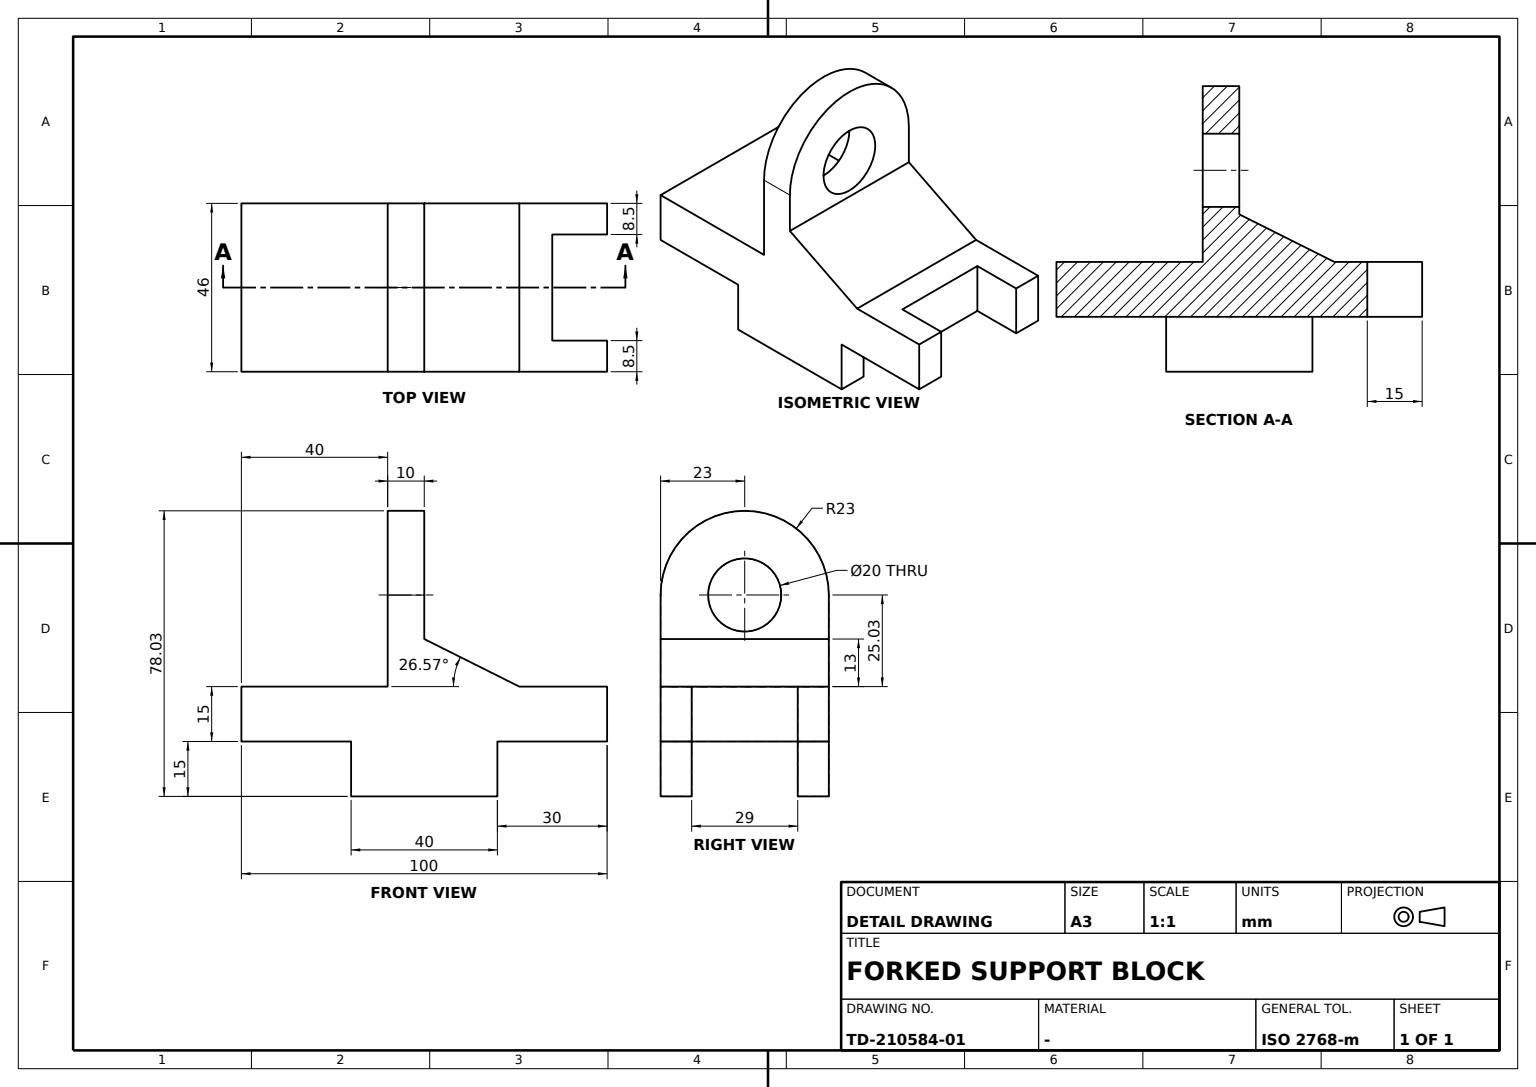
ISO-10303-21;
HEADER;
FILE_DESCRIPTION((''),'2;1');
FILE_NAME('','',(''),(''),'','','');
FILE_SCHEMA(('AUTOMOTIVE_DESIGN'));
ENDSEC;
DATA;
#1=APPLICATION_CONTEXT('');
#2=PRODUCT_CONTEXT('',#1,'mechanical');
#3=PRODUCT('','','',(#2));
#4=PRODUCT_DEFINITION_FORMATION('','',#3);
#5=PRODUCT_DEFINITION_CONTEXT('',#1,'design');
#6=PRODUCT_DEFINITION('','',#4,#5);
#7=PRODUCT_DEFINITION_SHAPE('','',#6);
#8=(LENGTH_UNIT()NAMED_UNIT(*)SI_UNIT(.MILLI.,.METRE.));
#9=(NAMED_UNIT(*)PLANE_ANGLE_UNIT()SI_UNIT($,.RADIAN.));
#10=(NAMED_UNIT(*)SI_UNIT($,.STERADIAN.)SOLID_ANGLE_UNIT());
#11=UNCERTAINTY_MEASURE_WITH_UNIT(LENGTH_MEASURE(1.E-05),#8,'distance_accuracy_value','');
#12=(GEOMETRIC_REPRESENTATION_CONTEXT(3)GLOBAL_UNCERTAINTY_ASSIGNED_CONTEXT((#11))GLOBAL_UNIT_ASSIGNED_CONTEXT((#8,#9,#10))REPRESENTATION_CONTEXT('',''));
#13=CARTESIAN_POINT('',(-20.,14.5,0.));
#14=VERTEX_POINT('',#13);
#15=CARTESIAN_POINT('',(-20.,23.,0.));
#16=VERTEX_POINT('',#15);
#17=CARTESIAN_POINT('',(-20.,18.75,0.));
#18=DIRECTION('',(0.,1.,0.));
#19=VECTOR('',#18,1000.);
#20=LINE('',#17,#19);
#21=EDGE_CURVE('',#14,#16,#20,.T.);
#22=ORIENTED_EDGE('',*,*,#21,.T.);
#23=CARTESIAN_POINT('',(20.,23.,0.));
#24=VERTEX_POINT('',#23);
#25=CARTESIAN_POINT('',(0.,23.,0.));
#26=DIRECTION('',(-1.,0.,0.));
#27=VECTOR('',#26,1000.);
#28=LINE('',#25,#27);
#29=EDGE_CURVE('',#24,#16,#28,.T.);
#30=ORIENTED_EDGE('',*,*,#29,.F.);
#31=CARTESIAN_POINT('',(20.,14.5,0.));
#32=VERTEX_POINT('',#31);
#33=CARTESIAN_POINT('',(20.,18.75,0.));
#34=LINE('',#33,#19);
#35=EDGE_CURVE('',#32,#24,#34,.T.);
#36=ORIENTED_EDGE('',*,*,#35,.F.);
#37=CARTESIAN_POINT('',(0.,14.5,0.));
#38=DIRECTION('',(1.,0.,0.));
#39=VECTOR('',#38,1000.);
#40=LINE('',#37,#39);
#41=EDGE_CURVE('',#14,#32,#40,.T.);
#42=ORIENTED_EDGE('',*,*,#41,.F.);
#43=EDGE_LOOP('',(#22,#30,#36,#42));
#44=FACE_OUTER_BOUND('',#43,.T.);
#45=CARTESIAN_POINT('',(20.,0.,0.));
#46=DIRECTION('',(0.,0.,-1.));
#47=AXIS2_PLACEMENT_3D('',#45,#46,#26);
#48=PLANE('',#47);
#49=ADVANCED_FACE('',(#44),#48,.T.);
#50=CARTESIAN_POINT('',(-20.,14.5,15.));
#51=VERTEX_POINT('',#50);
#52=CARTESIAN_POINT('',(-20.,23.,15.));
#53=VERTEX_POINT('',#52);
#54=CARTESIAN_POINT('',(-20.,18.75,15.));
#55=LINE('',#54,#19);
#56=EDGE_CURVE('',#51,#53,#55,.T.);
#57=ORIENTED_EDGE('',*,*,#56,.T.);
#58=CARTESIAN_POINT('',(-20.,23.,7.5));
#59=DIRECTION('',(0.,0.,1.));
#60=VECTOR('',#59,1000.);
#61=LINE('',#58,#60);
#62=EDGE_CURVE('',#16,#53,#61,.T.);
#63=ORIENTED_EDGE('',*,*,#62,.F.);
#64=ORIENTED_EDGE('',*,*,#21,.F.);
#65=CARTESIAN_POINT('',(-20.,14.5,7.5));
#66=VECTOR('',#46,1000.);
#67=LINE('',#65,#66);
#68=EDGE_CURVE('',#51,#14,#67,.T.);
#69=ORIENTED_EDGE('',*,*,#68,.F.);
#70=EDGE_LOOP('',(#57,#63,#64,#69));
#71=FACE_OUTER_BOUND('',#70,.T.);
#72=CARTESIAN_POINT('',(-20.,0.,0.));
#73=AXIS2_PLACEMENT_3D('',#72,#26,#59);
#74=PLANE('',#73);
#75=ADVANCED_FACE('',(#71),#74,.T.);
#76=CARTESIAN_POINT('',(50.,14.5,15.));
#77=VERTEX_POINT('',#76);
#78=CARTESIAN_POINT('',(50.,23.,15.));
#79=VERTEX_POINT('',#78);
#80=CARTESIAN_POINT('',(50.,18.75,15.));
#81=LINE('',#80,#19);
#82=EDGE_CURVE('',#77,#79,#81,.T.);
#83=ORIENTED_EDGE('',*,*,#82,.T.);
#84=CARTESIAN_POINT('',(50.,23.,30.));
#85=VERTEX_POINT('',#84);
#86=CARTESIAN_POINT('',(50.,23.,22.5));
#87=LINE('',#86,#66);
#88=EDGE_CURVE('',#85,#79,#87,.T.);
#89=ORIENTED_EDGE('',*,*,#88,.F.);
#90=CARTESIAN_POINT('',(50.,14.5,30.));
#91=VERTEX_POINT('',#90);
#92=CARTESIAN_POINT('',(50.,18.75,30.));
#93=LINE('',#92,#19);
#94=EDGE_CURVE('',#91,#85,#93,.T.);
#95=ORIENTED_EDGE('',*,*,#94,.F.);
#96=CARTESIAN_POINT('',(50.,14.5,22.5));
#97=LINE('',#96,#66);
#98=EDGE_CURVE('',#91,#77,#97,.T.);
#99=ORIENTED_EDGE('',*,*,#98,.T.);
#100=EDGE_LOOP('',(#83,#89,#95,#99));
#101=FACE_OUTER_BOUND('',#100,.T.);
#102=CARTESIAN_POINT('',(50.,0.,15.));
#103=AXIS2_PLACEMENT_3D('',#102,#26,#59);
#104=PLANE('',#103);
#105=ADVANCED_FACE('',(#101),#104,.F.);
#106=CARTESIAN_POINT('',(-10.,23.,55.034304));
#107=VERTEX_POINT('',#106);
#108=CARTESIAN_POINT('',(-10.,-23.,55.034304));
#109=VERTEX_POINT('',#108);
#110=CARTESIAN_POINT('',(-10.,0.,55.034304));
#111=AXIS2_PLACEMENT_3D('',#110,#38,#18);
#112=CIRCLE('',#111,23.);
#113=EDGE_CURVE('',#107,#109,#112,.T.);
#114=ORIENTED_EDGE('',*,*,#113,.F.);
#115=CARTESIAN_POINT('',(-10.,23.,55.));
#116=VERTEX_POINT('',#115);
#117=EDGE_CURVE('',#116,#107,#112,.T.);
#118=ORIENTED_EDGE('',*,*,#117,.F.);
#119=CARTESIAN_POINT('',(-10.,23.,30.));
#120=VERTEX_POINT('',#119);
#121=CARTESIAN_POINT('',(-10.,23.,42.5));
#122=LINE('',#121,#60);
#123=EDGE_CURVE('',#120,#116,#122,.T.);
#124=ORIENTED_EDGE('',*,*,#123,.F.);
#125=CARTESIAN_POINT('',(-10.,-23.,30.));
#126=VERTEX_POINT('',#125);
#127=CARTESIAN_POINT('',(-10.,0.,30.));
#128=LINE('',#127,#19);
#129=EDGE_CURVE('',#126,#120,#128,.T.);
#130=ORIENTED_EDGE('',*,*,#129,.F.);
#131=CARTESIAN_POINT('',(-10.,-22.999974,55.));
#132=VERTEX_POINT('',#131);
#133=CARTESIAN_POINT('',(-10.,-23.,42.5));
#134=LINE('',#133,#60);
#135=EDGE_CURVE('',#126,#132,#134,.T.);
#136=ORIENTED_EDGE('',*,*,#135,.T.);
#137=EDGE_CURVE('',#109,#132,#112,.T.);
#138=ORIENTED_EDGE('',*,*,#137,.F.);
#139=EDGE_LOOP('',(#114,#118,#124,#130,#136,#138));
#140=FACE_OUTER_BOUND('',#139,.T.);
#141=CARTESIAN_POINT('',(-10.,-10.,55.034304));
#142=VERTEX_POINT('',#141);
#143=CARTESIAN_POINT('',(-10.,10.,55.034304));
#144=VERTEX_POINT('',#143);
#145=CIRCLE('',#111,10.);
#146=EDGE_CURVE('',#142,#144,#145,.T.);
#147=ORIENTED_EDGE('',*,*,#146,.T.);
#148=EDGE_CURVE('',#144,#142,#145,.T.);
#149=ORIENTED_EDGE('',*,*,#148,.T.);
#150=EDGE_LOOP('',(#147,#149));
#151=FACE_BOUND('',#150,.T.);
#152=AXIS2_PLACEMENT_3D('',#127,#26,#59);
#153=PLANE('',#152);
#154=ADVANCED_FACE('',(#140,#151),#153,.T.);
#155=CARTESIAN_POINT('',(-20.,-14.5,0.));
#156=VERTEX_POINT('',#155);
#157=CARTESIAN_POINT('',(20.,-14.5,0.));
#158=VERTEX_POINT('',#157);
#159=CARTESIAN_POINT('',(0.,-14.5,0.));
#160=LINE('',#159,#39);
#161=EDGE_CURVE('',#156,#158,#160,.T.);
#162=ORIENTED_EDGE('',*,*,#161,.F.);
#163=CARTESIAN_POINT('',(-20.,-14.5,15.));
#164=VERTEX_POINT('',#163);
#165=CARTESIAN_POINT('',(-20.,-14.5,7.5));
#166=LINE('',#165,#60);
#167=EDGE_CURVE('',#156,#164,#166,.T.);
#168=ORIENTED_EDGE('',*,*,#167,.T.);
#169=CARTESIAN_POINT('',(20.,-14.5,15.));
#170=VERTEX_POINT('',#169);
#171=CARTESIAN_POINT('',(0.,-14.5,15.));
#172=LINE('',#171,#39);
#173=EDGE_CURVE('',#164,#170,#172,.T.);
#174=ORIENTED_EDGE('',*,*,#173,.T.);
#175=CARTESIAN_POINT('',(20.,-14.5,7.5));
#176=LINE('',#175,#66);
#177=EDGE_CURVE('',#170,#158,#176,.T.);
#178=ORIENTED_EDGE('',*,*,#177,.T.);
#179=EDGE_LOOP('',(#162,#168,#174,#178));
#180=FACE_OUTER_BOUND('',#179,.T.);
#181=DIRECTION('',(0.,-1.,0.));
#182=AXIS2_PLACEMENT_3D('',#163,#181,#46);
#183=PLANE('',#182);
#184=ADVANCED_FACE('',(#180),#183,.F.);
#185=CARTESIAN_POINT('',(35.,14.5,15.));
#186=VERTEX_POINT('',#185);
#187=CARTESIAN_POINT('',(42.5,14.5,15.));
#188=LINE('',#187,#27);
#189=EDGE_CURVE('',#77,#186,#188,.T.);
#190=ORIENTED_EDGE('',*,*,#189,.F.);
#191=ORIENTED_EDGE('',*,*,#98,.F.);
#192=CARTESIAN_POINT('',(35.,14.5,30.));
#193=VERTEX_POINT('',#192);
#194=CARTESIAN_POINT('',(42.5,14.5,30.));
#195=LINE('',#194,#27);
#196=EDGE_CURVE('',#91,#193,#195,.T.);
#197=ORIENTED_EDGE('',*,*,#196,.T.);
#198=CARTESIAN_POINT('',(35.,14.5,22.5));
#199=LINE('',#198,#66);
#200=EDGE_CURVE('',#193,#186,#199,.T.);
#201=ORIENTED_EDGE('',*,*,#200,.T.);
#202=EDGE_LOOP('',(#190,#191,#197,#201));
#203=FACE_OUTER_BOUND('',#202,.T.);
#204=AXIS2_PLACEMENT_3D('',#13,#18,#59);
#205=PLANE('',#204);
#206=ADVANCED_FACE('',(#203),#205,.F.);
#207=CARTESIAN_POINT('',(0.,23.,55.034304));
#208=VERTEX_POINT('',#207);
#209=CARTESIAN_POINT('',(-5.,23.,55.034304));
#210=LINE('',#209,#27);
#211=EDGE_CURVE('',#208,#107,#210,.T.);
#212=ORIENTED_EDGE('',*,*,#211,.T.);
#213=ORIENTED_EDGE('',*,*,#113,.T.);
#214=CARTESIAN_POINT('',(0.,-23.,55.034304));
#215=VERTEX_POINT('',#214);
#216=CARTESIAN_POINT('',(-5.,-23.,55.034304));
#217=LINE('',#216,#27);
#218=EDGE_CURVE('',#215,#109,#217,.T.);
#219=ORIENTED_EDGE('',*,*,#218,.F.);
#220=CARTESIAN_POINT('',(0.,0.,55.034304));
#221=AXIS2_PLACEMENT_3D('',#220,#38,#18);
#222=CIRCLE('',#221,23.);
#223=EDGE_CURVE('',#208,#215,#222,.T.);
#224=ORIENTED_EDGE('',*,*,#223,.F.);
#225=EDGE_LOOP('',(#212,#213,#219,#224));
#226=FACE_OUTER_BOUND('',#225,.T.);
#227=CARTESIAN_POINT('',(-5.,0.,55.034304));
#228=AXIS2_PLACEMENT_3D('',#227,#26,#18);
#229=CYLINDRICAL_SURFACE('',#228,23.);
#230=ADVANCED_FACE('',(#226),#229,.T.);
#231=CARTESIAN_POINT('',(20.,-23.,0.));
#232=VERTEX_POINT('',#231);
#233=CARTESIAN_POINT('',(20.,-18.75,0.));
#234=LINE('',#233,#19);
#235=EDGE_CURVE('',#232,#158,#234,.T.);
#236=ORIENTED_EDGE('',*,*,#235,.F.);
#237=CARTESIAN_POINT('',(-20.,-23.,0.));
#238=VERTEX_POINT('',#237);
#239=CARTESIAN_POINT('',(0.,-23.,0.));
#240=LINE('',#239,#27);
#241=EDGE_CURVE('',#232,#238,#240,.T.);
#242=ORIENTED_EDGE('',*,*,#241,.T.);
#243=CARTESIAN_POINT('',(-20.,-18.75,0.));
#244=LINE('',#243,#19);
#245=EDGE_CURVE('',#238,#156,#244,.T.);
#246=ORIENTED_EDGE('',*,*,#245,.T.);
#247=ORIENTED_EDGE('',*,*,#161,.T.);
#248=EDGE_LOOP('',(#236,#242,#246,#247));
#249=FACE_OUTER_BOUND('',#248,.T.);
#250=ADVANCED_FACE('',(#249),#48,.T.);
#251=ORIENTED_EDGE('',*,*,#173,.F.);
#252=CARTESIAN_POINT('',(-20.,-23.,15.));
#253=VERTEX_POINT('',#252);
#254=CARTESIAN_POINT('',(-20.,-18.75,15.));
#255=LINE('',#254,#19);
#256=EDGE_CURVE('',#253,#164,#255,.T.);
#257=ORIENTED_EDGE('',*,*,#256,.F.);
#258=CARTESIAN_POINT('',(-50.,-23.,15.));
#259=VERTEX_POINT('',#258);
#260=CARTESIAN_POINT('',(-35.,-23.,15.));
#261=LINE('',#260,#27);
#262=EDGE_CURVE('',#253,#259,#261,.T.);
#263=ORIENTED_EDGE('',*,*,#262,.T.);
#264=CARTESIAN_POINT('',(-50.,23.,15.));
#265=VERTEX_POINT('',#264);
#266=CARTESIAN_POINT('',(-50.,0.,15.));
#267=LINE('',#266,#19);
#268=EDGE_CURVE('',#259,#265,#267,.T.);
#269=ORIENTED_EDGE('',*,*,#268,.T.);
#270=CARTESIAN_POINT('',(-35.,23.,15.));
#271=LINE('',#270,#27);
#272=EDGE_CURVE('',#53,#265,#271,.T.);
#273=ORIENTED_EDGE('',*,*,#272,.F.);
#274=ORIENTED_EDGE('',*,*,#56,.F.);
#275=CARTESIAN_POINT('',(20.,14.5,15.));
#276=VERTEX_POINT('',#275);
#277=CARTESIAN_POINT('',(0.,14.5,15.));
#278=LINE('',#277,#39);
#279=EDGE_CURVE('',#51,#276,#278,.T.);
#280=ORIENTED_EDGE('',*,*,#279,.T.);
#281=CARTESIAN_POINT('',(20.,23.,15.));
#282=VERTEX_POINT('',#281);
#283=CARTESIAN_POINT('',(20.,18.75,15.));
#284=LINE('',#283,#19);
#285=EDGE_CURVE('',#276,#282,#284,.T.);
#286=ORIENTED_EDGE('',*,*,#285,.T.);
#287=CARTESIAN_POINT('',(35.,23.,15.));
#288=LINE('',#287,#27);
#289=EDGE_CURVE('',#79,#282,#288,.T.);
#290=ORIENTED_EDGE('',*,*,#289,.F.);
#291=ORIENTED_EDGE('',*,*,#82,.F.);
#292=ORIENTED_EDGE('',*,*,#189,.T.);
#293=CARTESIAN_POINT('',(35.,-14.5,15.));
#294=VERTEX_POINT('',#293);
#295=CARTESIAN_POINT('',(35.,0.,15.));
#296=LINE('',#295,#19);
#297=EDGE_CURVE('',#294,#186,#296,.T.);
#298=ORIENTED_EDGE('',*,*,#297,.F.);
#299=CARTESIAN_POINT('',(50.,-14.5,15.));
#300=VERTEX_POINT('',#299);
#301=CARTESIAN_POINT('',(42.5,-14.5,15.));
#302=LINE('',#301,#27);
#303=EDGE_CURVE('',#300,#294,#302,.T.);
#304=ORIENTED_EDGE('',*,*,#303,.F.);
#305=CARTESIAN_POINT('',(50.,-23.,15.));
#306=VERTEX_POINT('',#305);
#307=CARTESIAN_POINT('',(50.,-18.75,15.));
#308=LINE('',#307,#19);
#309=EDGE_CURVE('',#306,#300,#308,.T.);
#310=ORIENTED_EDGE('',*,*,#309,.F.);
#311=CARTESIAN_POINT('',(20.,-23.,15.));
#312=VERTEX_POINT('',#311);
#313=CARTESIAN_POINT('',(35.,-23.,15.));
#314=LINE('',#313,#27);
#315=EDGE_CURVE('',#306,#312,#314,.T.);
#316=ORIENTED_EDGE('',*,*,#315,.T.);
#317=CARTESIAN_POINT('',(20.,-18.75,15.));
#318=LINE('',#317,#19);
#319=EDGE_CURVE('',#312,#170,#318,.T.);
#320=ORIENTED_EDGE('',*,*,#319,.T.);
#321=EDGE_LOOP('',(#251,#257,#263,#269,#273,#274,#280,#286,#290,#291,#292,#298,#304,#310,#316,#320));
#322=FACE_OUTER_BOUND('',#321,.T.);
#323=CARTESIAN_POINT('',(-20.,0.,15.));
#324=AXIS2_PLACEMENT_3D('',#323,#46,#26);
#325=PLANE('',#324);
#326=ADVANCED_FACE('',(#322),#325,.T.);
#327=ORIENTED_EDGE('',*,*,#41,.T.);
#328=CARTESIAN_POINT('',(20.,14.5,7.5));
#329=LINE('',#328,#60);
#330=EDGE_CURVE('',#32,#276,#329,.T.);
#331=ORIENTED_EDGE('',*,*,#330,.T.);
#332=ORIENTED_EDGE('',*,*,#279,.F.);
#333=ORIENTED_EDGE('',*,*,#68,.T.);
#334=EDGE_LOOP('',(#327,#331,#332,#333));
#335=FACE_OUTER_BOUND('',#334,.T.);
#336=ADVANCED_FACE('',(#335),#205,.F.);
#337=CARTESIAN_POINT('',(-50.,23.,30.));
#338=VERTEX_POINT('',#337);
#339=CARTESIAN_POINT('',(-30.,23.,30.));
#340=LINE('',#339,#39);
#341=EDGE_CURVE('',#338,#120,#340,.T.);
#342=ORIENTED_EDGE('',*,*,#341,.T.);
#343=ORIENTED_EDGE('',*,*,#123,.T.);
#344=CARTESIAN_POINT('',(0.,22.999974,55.));
#345=VERTEX_POINT('',#344);
#346=CARTESIAN_POINT('',(-6.666667,23.,55.));
#347=CARTESIAN_POINT('',(-3.333333,23.,55.));
#348=B_SPLINE_CURVE_WITH_KNOTS('',3,(#115,#346,#347,#344),.UNSPECIFIED.,.F.,.F.,(4,4),(0.,1.),.UNSPECIFIED.);
#349=EDGE_CURVE('',#116,#345,#348,.T.);
#350=ORIENTED_EDGE('',*,*,#349,.T.);
#351=CARTESIAN_POINT('',(0.,23.,43.));
#352=VERTEX_POINT('',#351);
#353=CARTESIAN_POINT('',(0.,23.,49.));
#354=LINE('',#353,#66);
#355=EDGE_CURVE('',#345,#352,#354,.T.);
#356=ORIENTED_EDGE('',*,*,#355,.T.);
#357=CARTESIAN_POINT('',(26.,23.,30.));
#358=VERTEX_POINT('',#357);
#359=CARTESIAN_POINT('',(13.,23.,36.5));
#360=DIRECTION('',(0.894427191,0.,-0.447213595));
#361=VECTOR('',#360,1000.);
#362=LINE('',#359,#361);
#363=EDGE_CURVE('',#352,#358,#362,.T.);
#364=ORIENTED_EDGE('',*,*,#363,.T.);
#365=CARTESIAN_POINT('',(38.,23.,30.));
#366=LINE('',#365,#39);
#367=EDGE_CURVE('',#358,#85,#366,.T.);
#368=ORIENTED_EDGE('',*,*,#367,.T.);
#369=ORIENTED_EDGE('',*,*,#88,.T.);
#370=ORIENTED_EDGE('',*,*,#289,.T.);
#371=CARTESIAN_POINT('',(20.,23.,7.5));
#372=LINE('',#371,#66);
#373=EDGE_CURVE('',#282,#24,#372,.T.);
#374=ORIENTED_EDGE('',*,*,#373,.T.);
#375=ORIENTED_EDGE('',*,*,#29,.T.);
#376=ORIENTED_EDGE('',*,*,#62,.T.);
#377=ORIENTED_EDGE('',*,*,#272,.T.);
#378=CARTESIAN_POINT('',(-50.,23.,22.5));
#379=LINE('',#378,#60);
#380=EDGE_CURVE('',#265,#338,#379,.T.);
#381=ORIENTED_EDGE('',*,*,#380,.T.);
#382=EDGE_LOOP('',(#342,#343,#350,#356,#364,#368,#369,#370,#374,#375,#376,#377,#381));
#383=FACE_OUTER_BOUND('',#382,.T.);
#384=AXIS2_PLACEMENT_3D('',#25,#18,#26);
#385=PLANE('',#384);
#386=ADVANCED_FACE('',(#383),#385,.T.);
#387=ORIENTED_EDGE('',*,*,#148,.F.);
#388=CARTESIAN_POINT('',(0.,10.,55.034304));
#389=VERTEX_POINT('',#388);
#390=CARTESIAN_POINT('',(-5.,10.,55.034304));
#391=LINE('',#390,#27);
#392=EDGE_CURVE('',#389,#144,#391,.T.);
#393=ORIENTED_EDGE('',*,*,#392,.F.);
#394=CARTESIAN_POINT('',(0.,-10.,55.034304));
#395=VERTEX_POINT('',#394);
#396=CIRCLE('',#221,10.);
#397=EDGE_CURVE('',#389,#395,#396,.T.);
#398=ORIENTED_EDGE('',*,*,#397,.T.);
#399=CARTESIAN_POINT('',(-5.,-10.,55.034304));
#400=LINE('',#399,#27);
#401=EDGE_CURVE('',#395,#142,#400,.T.);
#402=ORIENTED_EDGE('',*,*,#401,.T.);
#403=EDGE_LOOP('',(#387,#393,#398,#402));
#404=FACE_OUTER_BOUND('',#403,.T.);
#405=CYLINDRICAL_SURFACE('',#228,10.);
#406=ADVANCED_FACE('',(#404),#405,.F.);
#407=CARTESIAN_POINT('',(-50.,-23.,30.));
#408=VERTEX_POINT('',#407);
#409=CARTESIAN_POINT('',(-30.,-23.,30.));
#410=LINE('',#409,#39);
#411=EDGE_CURVE('',#408,#126,#410,.T.);
#412=ORIENTED_EDGE('',*,*,#411,.T.);
#413=ORIENTED_EDGE('',*,*,#129,.T.);
#414=ORIENTED_EDGE('',*,*,#341,.F.);
#415=CARTESIAN_POINT('',(-50.,0.,30.));
#416=LINE('',#415,#19);
#417=EDGE_CURVE('',#408,#338,#416,.T.);
#418=ORIENTED_EDGE('',*,*,#417,.F.);
#419=EDGE_LOOP('',(#412,#413,#414,#418));
#420=FACE_OUTER_BOUND('',#419,.T.);
#421=AXIS2_PLACEMENT_3D('',#415,#59,#38);
#422=PLANE('',#421);
#423=ADVANCED_FACE('',(#420),#422,.T.);
#424=CARTESIAN_POINT('',(0.,-23.,55.));
#425=VERTEX_POINT('',#424);
#426=EDGE_CURVE('',#215,#425,#222,.T.);
#427=ORIENTED_EDGE('',*,*,#426,.T.);
#428=CARTESIAN_POINT('',(0.,-23.,43.));
#429=VERTEX_POINT('',#428);
#430=CARTESIAN_POINT('',(0.,-23.,49.));
#431=LINE('',#430,#66);
#432=EDGE_CURVE('',#425,#429,#431,.T.);
#433=ORIENTED_EDGE('',*,*,#432,.T.);
#434=CARTESIAN_POINT('',(0.,0.,43.));
#435=LINE('',#434,#19);
#436=EDGE_CURVE('',#429,#352,#435,.T.);
#437=ORIENTED_EDGE('',*,*,#436,.T.);
#438=ORIENTED_EDGE('',*,*,#355,.F.);
#439=EDGE_CURVE('',#345,#208,#222,.T.);
#440=ORIENTED_EDGE('',*,*,#439,.T.);
#441=ORIENTED_EDGE('',*,*,#223,.T.);
#442=EDGE_LOOP('',(#427,#433,#437,#438,#440,#441));
#443=FACE_OUTER_BOUND('',#442,.T.);
#444=ORIENTED_EDGE('',*,*,#397,.F.);
#445=EDGE_CURVE('',#395,#389,#396,.T.);
#446=ORIENTED_EDGE('',*,*,#445,.F.);
#447=EDGE_LOOP('',(#444,#446));
#448=FACE_BOUND('',#447,.T.);
#449=CARTESIAN_POINT('',(0.,0.,55.));
#450=AXIS2_PLACEMENT_3D('',#449,#38,#46);
#451=PLANE('',#450);
#452=ADVANCED_FACE('',(#443,#448),#451,.T.);
#453=ORIENTED_EDGE('',*,*,#200,.F.);
#454=CARTESIAN_POINT('',(35.,-14.5,30.));
#455=VERTEX_POINT('',#454);
#456=CARTESIAN_POINT('',(35.,0.,30.));
#457=VECTOR('',#181,1000.);
#458=LINE('',#456,#457);
#459=EDGE_CURVE('',#193,#455,#458,.T.);
#460=ORIENTED_EDGE('',*,*,#459,.T.);
#461=CARTESIAN_POINT('',(35.,-14.5,22.5));
#462=LINE('',#461,#66);
#463=EDGE_CURVE('',#455,#294,#462,.T.);
#464=ORIENTED_EDGE('',*,*,#463,.T.);
#465=ORIENTED_EDGE('',*,*,#297,.T.);
#466=EDGE_LOOP('',(#453,#460,#464,#465));
#467=FACE_OUTER_BOUND('',#466,.T.);
#468=AXIS2_PLACEMENT_3D('',#454,#26,#18);
#469=PLANE('',#468);
#470=ADVANCED_FACE('',(#467),#469,.F.);
#471=ORIENTED_EDGE('',*,*,#285,.F.);
#472=ORIENTED_EDGE('',*,*,#330,.F.);
#473=ORIENTED_EDGE('',*,*,#35,.T.);
#474=ORIENTED_EDGE('',*,*,#373,.F.);
#475=EDGE_LOOP('',(#471,#472,#473,#474));
#476=FACE_OUTER_BOUND('',#475,.T.);
#477=AXIS2_PLACEMENT_3D('',#45,#26,#59);
#478=PLANE('',#477);
#479=ADVANCED_FACE('',(#476),#478,.F.);
#480=CARTESIAN_POINT('',(-20.,-23.,7.5));
#481=LINE('',#480,#60);
#482=EDGE_CURVE('',#238,#253,#481,.T.);
#483=ORIENTED_EDGE('',*,*,#482,.F.);
#484=ORIENTED_EDGE('',*,*,#241,.F.);
#485=CARTESIAN_POINT('',(20.,-23.,7.5));
#486=LINE('',#485,#66);
#487=EDGE_CURVE('',#312,#232,#486,.T.);
#488=ORIENTED_EDGE('',*,*,#487,.F.);
#489=ORIENTED_EDGE('',*,*,#315,.F.);
#490=CARTESIAN_POINT('',(50.,-23.,30.));
#491=VERTEX_POINT('',#490);
#492=CARTESIAN_POINT('',(50.,-23.,22.5));
#493=LINE('',#492,#66);
#494=EDGE_CURVE('',#491,#306,#493,.T.);
#495=ORIENTED_EDGE('',*,*,#494,.F.);
#496=CARTESIAN_POINT('',(26.,-23.,30.));
#497=VERTEX_POINT('',#496);
#498=CARTESIAN_POINT('',(38.,-23.,30.));
#499=LINE('',#498,#39);
#500=EDGE_CURVE('',#497,#491,#499,.T.);
#501=ORIENTED_EDGE('',*,*,#500,.F.);
#502=CARTESIAN_POINT('',(13.,-23.,36.5));
#503=LINE('',#502,#361);
#504=EDGE_CURVE('',#429,#497,#503,.T.);
#505=ORIENTED_EDGE('',*,*,#504,.F.);
#506=ORIENTED_EDGE('',*,*,#432,.F.);
#507=CARTESIAN_POINT('',(-6.666667,-22.999974,55.));
#508=CARTESIAN_POINT('',(-3.333333,-22.999974,55.));
#509=B_SPLINE_CURVE_WITH_KNOTS('',3,(#131,#507,#508,#424),.UNSPECIFIED.,.F.,.F.,(4,4),(0.,1.),.UNSPECIFIED.);
#510=EDGE_CURVE('',#132,#425,#509,.T.);
#511=ORIENTED_EDGE('',*,*,#510,.F.);
#512=ORIENTED_EDGE('',*,*,#135,.F.);
#513=ORIENTED_EDGE('',*,*,#411,.F.);
#514=CARTESIAN_POINT('',(-50.,-23.,22.5));
#515=LINE('',#514,#60);
#516=EDGE_CURVE('',#259,#408,#515,.T.);
#517=ORIENTED_EDGE('',*,*,#516,.F.);
#518=ORIENTED_EDGE('',*,*,#262,.F.);
#519=EDGE_LOOP('',(#483,#484,#488,#489,#495,#501,#505,#506,#511,#512,#513,#517,#518));
#520=FACE_OUTER_BOUND('',#519,.T.);
#521=AXIS2_PLACEMENT_3D('',#239,#18,#26);
#522=PLANE('',#521);
#523=ADVANCED_FACE('',(#520),#522,.F.);
#524=ORIENTED_EDGE('',*,*,#516,.T.);
#525=ORIENTED_EDGE('',*,*,#417,.T.);
#526=ORIENTED_EDGE('',*,*,#380,.F.);
#527=ORIENTED_EDGE('',*,*,#268,.F.);
#528=EDGE_LOOP('',(#524,#525,#526,#527));
#529=FACE_OUTER_BOUND('',#528,.T.);
#530=AXIS2_PLACEMENT_3D('',#266,#26,#59);
#531=PLANE('',#530);
#532=ADVANCED_FACE('',(#529),#531,.T.);
#533=ORIENTED_EDGE('',*,*,#218,.T.);
#534=ORIENTED_EDGE('',*,*,#137,.T.);
#535=ORIENTED_EDGE('',*,*,#510,.T.);
#536=ORIENTED_EDGE('',*,*,#426,.F.);
#537=EDGE_LOOP('',(#533,#534,#535,#536));
#538=FACE_OUTER_BOUND('',#537,.T.);
#539=ADVANCED_FACE('',(#538),#229,.T.);
#540=ORIENTED_EDGE('',*,*,#494,.T.);
#541=ORIENTED_EDGE('',*,*,#309,.T.);
#542=CARTESIAN_POINT('',(50.,-14.5,30.));
#543=VERTEX_POINT('',#542);
#544=CARTESIAN_POINT('',(50.,-14.5,22.5));
#545=LINE('',#544,#66);
#546=EDGE_CURVE('',#543,#300,#545,.T.);
#547=ORIENTED_EDGE('',*,*,#546,.F.);
#548=CARTESIAN_POINT('',(50.,-18.75,30.));
#549=LINE('',#548,#19);
#550=EDGE_CURVE('',#491,#543,#549,.T.);
#551=ORIENTED_EDGE('',*,*,#550,.F.);
#552=EDGE_LOOP('',(#540,#541,#547,#551));
#553=FACE_OUTER_BOUND('',#552,.T.);
#554=ADVANCED_FACE('',(#553),#104,.F.);
#555=ORIENTED_EDGE('',*,*,#349,.F.);
#556=ORIENTED_EDGE('',*,*,#117,.T.);
#557=ORIENTED_EDGE('',*,*,#211,.F.);
#558=ORIENTED_EDGE('',*,*,#439,.F.);
#559=EDGE_LOOP('',(#555,#556,#557,#558));
#560=FACE_OUTER_BOUND('',#559,.T.);
#561=ADVANCED_FACE('',(#560),#229,.T.);
#562=ORIENTED_EDGE('',*,*,#235,.T.);
#563=ORIENTED_EDGE('',*,*,#177,.F.);
#564=ORIENTED_EDGE('',*,*,#319,.F.);
#565=ORIENTED_EDGE('',*,*,#487,.T.);
#566=EDGE_LOOP('',(#562,#563,#564,#565));
#567=FACE_OUTER_BOUND('',#566,.T.);
#568=ADVANCED_FACE('',(#567),#478,.F.);
#569=ORIENTED_EDGE('',*,*,#445,.T.);
#570=ORIENTED_EDGE('',*,*,#392,.T.);
#571=ORIENTED_EDGE('',*,*,#146,.F.);
#572=ORIENTED_EDGE('',*,*,#401,.F.);
#573=EDGE_LOOP('',(#569,#570,#571,#572));
#574=FACE_OUTER_BOUND('',#573,.T.);
#575=ADVANCED_FACE('',(#574),#405,.F.);
#576=CARTESIAN_POINT('',(26.,0.,30.));
#577=LINE('',#576,#19);
#578=EDGE_CURVE('',#497,#358,#577,.T.);
#579=ORIENTED_EDGE('',*,*,#578,.T.);
#580=ORIENTED_EDGE('',*,*,#363,.F.);
#581=ORIENTED_EDGE('',*,*,#436,.F.);
#582=ORIENTED_EDGE('',*,*,#504,.T.);
#583=EDGE_LOOP('',(#579,#580,#581,#582));
#584=FACE_OUTER_BOUND('',#583,.T.);
#585=DIRECTION('',(-0.447213595,0.,-0.894427191));
#586=DIRECTION('',(-0.894427191,0.,0.447213595));
#587=AXIS2_PLACEMENT_3D('',#576,#585,#586);
#588=PLANE('',#587);
#589=ADVANCED_FACE('',(#584),#588,.F.);
#590=ORIENTED_EDGE('',*,*,#196,.F.);
#591=ORIENTED_EDGE('',*,*,#94,.T.);
#592=ORIENTED_EDGE('',*,*,#367,.F.);
#593=ORIENTED_EDGE('',*,*,#578,.F.);
#594=ORIENTED_EDGE('',*,*,#500,.T.);
#595=ORIENTED_EDGE('',*,*,#550,.T.);
#596=CARTESIAN_POINT('',(42.5,-14.5,30.));
#597=LINE('',#596,#39);
#598=EDGE_CURVE('',#455,#543,#597,.T.);
#599=ORIENTED_EDGE('',*,*,#598,.F.);
#600=ORIENTED_EDGE('',*,*,#459,.F.);
#601=EDGE_LOOP('',(#590,#591,#592,#593,#594,#595,#599,#600));
#602=FACE_OUTER_BOUND('',#601,.T.);
#603=ADVANCED_FACE('',(#602),#422,.T.);
#604=ORIENTED_EDGE('',*,*,#303,.T.);
#605=ORIENTED_EDGE('',*,*,#463,.F.);
#606=ORIENTED_EDGE('',*,*,#598,.T.);
#607=ORIENTED_EDGE('',*,*,#546,.T.);
#608=EDGE_LOOP('',(#604,#605,#606,#607));
#609=FACE_OUTER_BOUND('',#608,.T.);
#610=ADVANCED_FACE('',(#609),#183,.F.);
#611=ORIENTED_EDGE('',*,*,#482,.T.);
#612=ORIENTED_EDGE('',*,*,#256,.T.);
#613=ORIENTED_EDGE('',*,*,#167,.F.);
#614=ORIENTED_EDGE('',*,*,#245,.F.);
#615=EDGE_LOOP('',(#611,#612,#613,#614));
#616=FACE_OUTER_BOUND('',#615,.T.);
#617=ADVANCED_FACE('',(#616),#74,.T.);
#618=CLOSED_SHELL('',(#49,#75,#105,#154,#184,#206,#230,#250,#326,#336,#386,#406,#423,#452,#470,#479,#523,#532,#539,#554,#561,#568,#575,#589,#603,#610,#617));
#619=MANIFOLD_SOLID_BREP('',#618);
#620=ADVANCED_BREP_SHAPE_REPRESENTATION('',(#619),#12);
#621=SHAPE_DEFINITION_REPRESENTATION(#7,#620);
ENDSEC;
END-ISO-10303-21;
